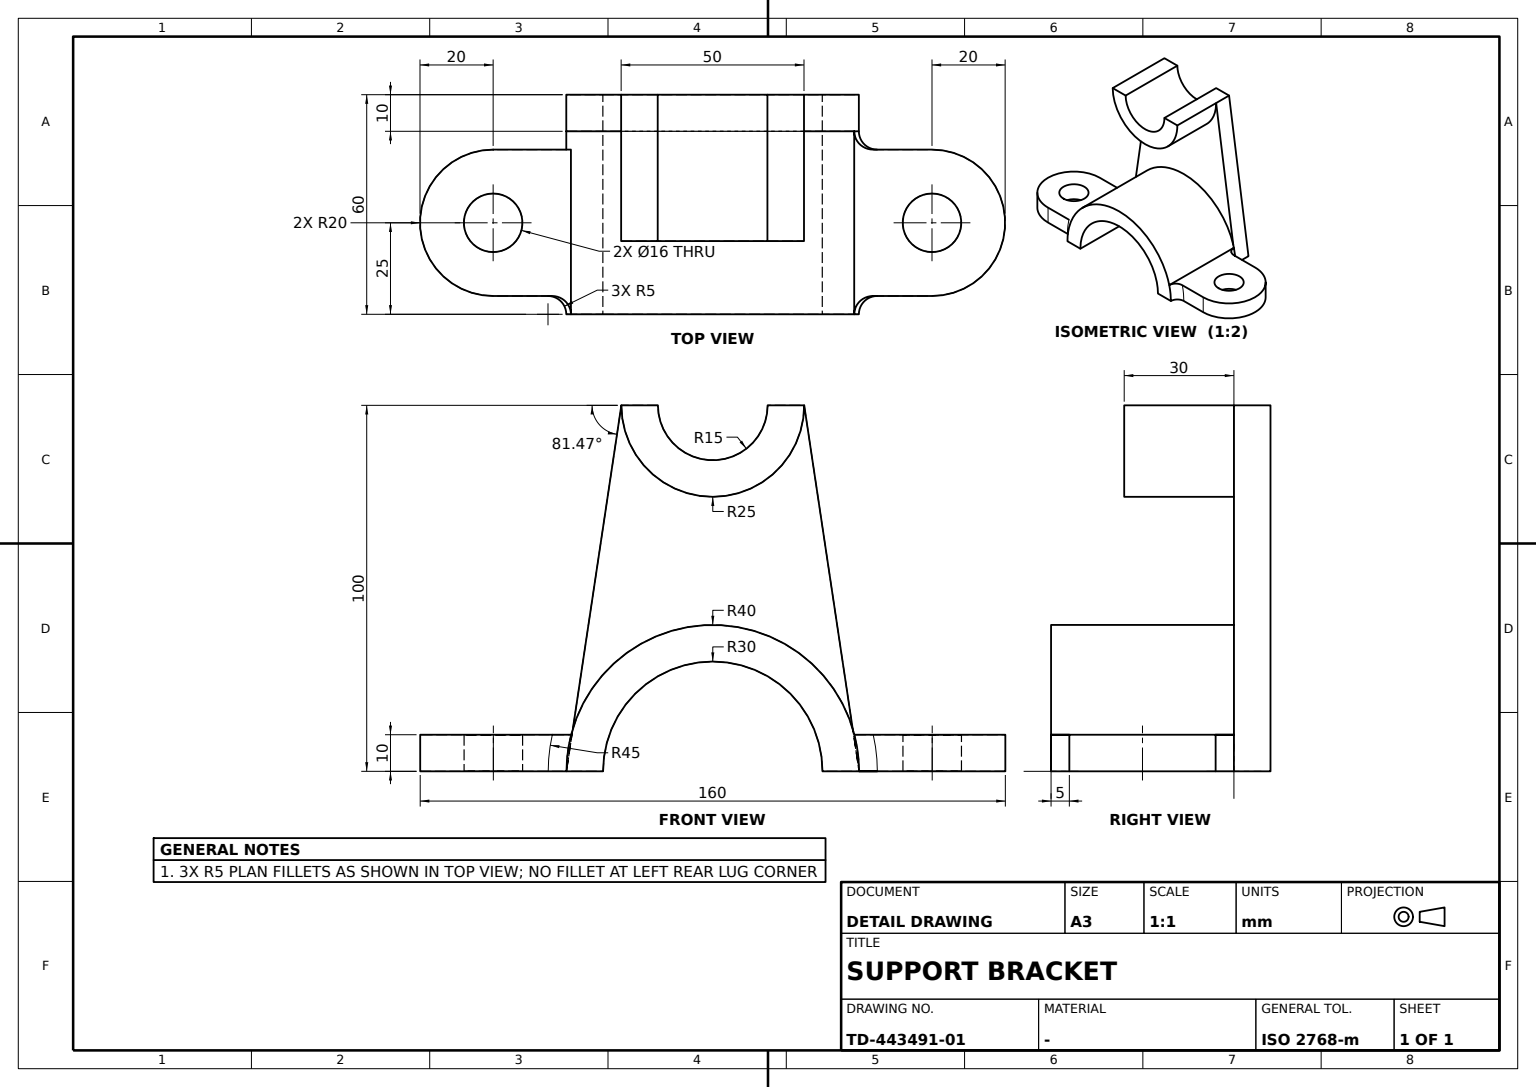
ISO-10303-21;
HEADER;
FILE_DESCRIPTION((''),'2;1');
FILE_NAME('','',(''),(''),'','','');
FILE_SCHEMA(('AUTOMOTIVE_DESIGN'));
ENDSEC;
DATA;
#1=APPLICATION_CONTEXT('');
#2=PRODUCT_CONTEXT('',#1,'mechanical');
#3=PRODUCT('','','',(#2));
#4=PRODUCT_DEFINITION_FORMATION('','',#3);
#5=PRODUCT_DEFINITION_CONTEXT('',#1,'design');
#6=PRODUCT_DEFINITION('','',#4,#5);
#7=PRODUCT_DEFINITION_SHAPE('','',#6);
#8=(LENGTH_UNIT()NAMED_UNIT(*)SI_UNIT(.MILLI.,.METRE.));
#9=(NAMED_UNIT(*)PLANE_ANGLE_UNIT()SI_UNIT($,.RADIAN.));
#10=(NAMED_UNIT(*)SI_UNIT($,.STERADIAN.)SOLID_ANGLE_UNIT());
#11=UNCERTAINTY_MEASURE_WITH_UNIT(LENGTH_MEASURE(0.005),#8,'distance_accuracy_value','');
#12=(GEOMETRIC_REPRESENTATION_CONTEXT(3)GLOBAL_UNCERTAINTY_ASSIGNED_CONTEXT((#11))GLOBAL_UNIT_ASSIGNED_CONTEXT((#8,#9,#10))REPRESENTATION_CONTEXT('',''));
#13=CARTESIAN_POINT('',(-8.,-60.,0.));
#14=VERTEX_POINT('',#13);
#15=CARTESIAN_POINT('',(0.,-60.,0.));
#16=DIRECTION('',(0.,0.,-1.));
#17=DIRECTION('',(-1.,0.,0.));
#18=AXIS2_PLACEMENT_3D('',#15,#16,#17);
#19=CIRCLE('',#18,8.);
#20=EDGE_CURVE('',#14,#14,#19,.T.);
#21=ORIENTED_EDGE('',*,*,#20,.T.);
#22=EDGE_LOOP('',(#21));
#23=FACE_BOUND('',#22,.T.);
#24=CARTESIAN_POINT('',(8.,-60.,10.));
#25=VERTEX_POINT('',#24);
#26=CARTESIAN_POINT('',(0.,-60.,10.));
#27=DIRECTION('',(0.,0.,1.));
#28=DIRECTION('',(1.,0.,0.));
#29=AXIS2_PLACEMENT_3D('',#26,#27,#28);
#30=CIRCLE('',#29,8.);
#31=EDGE_CURVE('',#25,#25,#30,.F.);
#32=ORIENTED_EDGE('',*,*,#31,.F.);
#33=EDGE_LOOP('',(#32));
#34=FACE_BOUND('',#33,.T.);
#35=CARTESIAN_POINT('',(0.,-60.,5.));
#36=AXIS2_PLACEMENT_3D('',#35,#16,#28);
#37=CYLINDRICAL_SURFACE('',#36,8.);
#38=ADVANCED_FACE('',(#23,#34),#37,.F.);
#39=CARTESIAN_POINT('',(20.,-45.,0.));
#40=VERTEX_POINT('',#39);
#41=CARTESIAN_POINT('',(25.,-40.,0.));
#42=VERTEX_POINT('',#41);
#43=CARTESIAN_POINT('',(25.,-45.,0.));
#44=AXIS2_PLACEMENT_3D('',#43,#16,#17);
#45=CIRCLE('',#44,5.);
#46=EDGE_CURVE('',#40,#42,#45,.T.);
#47=ORIENTED_EDGE('',*,*,#46,.F.);
#48=CARTESIAN_POINT('',(20.,-60.,0.));
#49=VERTEX_POINT('',#48);
#50=CARTESIAN_POINT('',(20.,40.,0.));
#51=DIRECTION('',(0.,-1.,0.));
#52=VECTOR('',#51,1000.);
#53=LINE('',#50,#52);
#54=EDGE_CURVE('',#40,#49,#53,.T.);
#55=ORIENTED_EDGE('',*,*,#54,.T.);
#56=CARTESIAN_POINT('',(-20.,-60.,0.));
#57=VERTEX_POINT('',#56);
#58=CIRCLE('',#18,20.);
#59=EDGE_CURVE('',#49,#57,#58,.T.);
#60=ORIENTED_EDGE('',*,*,#59,.T.);
#61=CARTESIAN_POINT('',(-20.,-40.,0.));
#62=VERTEX_POINT('',#61);
#63=CARTESIAN_POINT('',(-20.,40.,0.));
#64=DIRECTION('',(0.,1.,0.));
#65=VECTOR('',#64,1000.);
#66=LINE('',#63,#65);
#67=EDGE_CURVE('',#57,#62,#66,.T.);
#68=ORIENTED_EDGE('',*,*,#67,.T.);
#69=CARTESIAN_POINT('',(-25.,-40.,0.));
#70=VERTEX_POINT('',#69);
#71=VECTOR('',#17,1000.);
#72=LINE('',#61,#71);
#73=EDGE_CURVE('',#62,#70,#72,.T.);
#74=ORIENTED_EDGE('',*,*,#73,.T.);
#75=CARTESIAN_POINT('',(-35.,-40.,0.));
#76=VERTEX_POINT('',#75);
#77=LINE('',#69,#71);
#78=EDGE_CURVE('',#70,#76,#77,.T.);
#79=ORIENTED_EDGE('',*,*,#78,.T.);
#80=CARTESIAN_POINT('',(-35.,-30.,0.));
#81=VERTEX_POINT('',#80);
#82=CARTESIAN_POINT('',(-35.,0.,0.));
#83=LINE('',#82,#52);
#84=EDGE_CURVE('',#81,#76,#83,.T.);
#85=ORIENTED_EDGE('',*,*,#84,.F.);
#86=CARTESIAN_POINT('',(25.,-30.,0.));
#87=VERTEX_POINT('',#86);
#88=LINE('',#86,#71);
#89=EDGE_CURVE('',#87,#81,#88,.T.);
#90=ORIENTED_EDGE('',*,*,#89,.F.);
#91=CARTESIAN_POINT('',(25.,0.,0.));
#92=LINE('',#91,#52);
#93=EDGE_CURVE('',#87,#42,#92,.T.);
#94=ORIENTED_EDGE('',*,*,#93,.T.);
#95=EDGE_LOOP('',(#47,#55,#60,#68,#74,#79,#85,#90,#94));
#96=FACE_BOUND('',#95,.T.);
#97=ORIENTED_EDGE('',*,*,#20,.F.);
#98=EDGE_LOOP('',(#97));
#99=FACE_BOUND('',#98,.T.);
#100=CARTESIAN_POINT('',(0.,40.,0.));
#101=AXIS2_PLACEMENT_3D('',#100,#16,#51);
#102=PLANE('',#101);
#103=ADVANCED_FACE('',(#96,#99),#102,.T.);
#104=CARTESIAN_POINT('',(-25.,40.,0.));
#105=VERTEX_POINT('',#104);
#106=CARTESIAN_POINT('',(-25.,38.239609,11.735941));
#107=VERTEX_POINT('',#106);
#108=CARTESIAN_POINT('',(-25.,39.119804,5.867971));
#109=DIRECTION('',(0.,-0.148340453,0.988936353));
#110=VECTOR('',#109,1000.);
#111=LINE('',#108,#110);
#112=EDGE_CURVE('',#105,#107,#111,.T.);
#113=ORIENTED_EDGE('',*,*,#112,.T.);
#114=CARTESIAN_POINT('',(-25.,38.729833,10.));
#115=VERTEX_POINT('',#114);
#116=CARTESIAN_POINT('',(-25.,0.,0.));
#117=AXIS2_PLACEMENT_3D('',#116,#17,#27);
#118=CIRCLE('',#117,40.);
#119=EDGE_CURVE('',#107,#115,#118,.T.);
#120=ORIENTED_EDGE('',*,*,#119,.T.);
#121=EDGE_CURVE('',#115,#105,#118,.T.);
#122=ORIENTED_EDGE('',*,*,#121,.T.);
#123=EDGE_LOOP('',(#113,#120,#122));
#124=FACE_BOUND('',#123,.T.);
#125=AXIS2_PLACEMENT_3D('',#116,#17,#51);
#126=PLANE('',#125);
#127=ADVANCED_FACE('',(#124),#126,.T.);
#128=CARTESIAN_POINT('',(5.,-15.,100.));
#129=VERTEX_POINT('',#128);
#130=CARTESIAN_POINT('',(-35.,-15.,100.));
#131=VERTEX_POINT('',#130);
#132=VECTOR('',#28,1000.);
#133=LINE('',#128,#132);
#134=EDGE_CURVE('',#129,#131,#133,.F.);
#135=ORIENTED_EDGE('',*,*,#134,.T.);
#136=CARTESIAN_POINT('',(-35.,-25.,100.));
#137=VERTEX_POINT('',#136);
#138=CARTESIAN_POINT('',(-35.,0.,100.));
#139=LINE('',#138,#52);
#140=EDGE_CURVE('',#131,#137,#139,.T.);
#141=ORIENTED_EDGE('',*,*,#140,.T.);
#142=CARTESIAN_POINT('',(-25.,-25.,100.));
#143=VERTEX_POINT('',#142);
#144=LINE('',#142,#71);
#145=EDGE_CURVE('',#143,#137,#144,.T.);
#146=ORIENTED_EDGE('',*,*,#145,.F.);
#147=CARTESIAN_POINT('',(5.,-25.,100.));
#148=VERTEX_POINT('',#147);
#149=LINE('',#142,#132);
#150=EDGE_CURVE('',#143,#148,#149,.T.);
#151=ORIENTED_EDGE('',*,*,#150,.T.);
#152=CARTESIAN_POINT('',(5.,0.,100.));
#153=LINE('',#152,#65);
#154=EDGE_CURVE('',#148,#129,#153,.T.);
#155=ORIENTED_EDGE('',*,*,#154,.T.);
#156=EDGE_LOOP('',(#135,#141,#146,#151,#155));
#157=FACE_BOUND('',#156,.T.);
#158=CARTESIAN_POINT('',(-25.,25.,100.));
#159=AXIS2_PLACEMENT_3D('',#158,#16,#51);
#160=PLANE('',#159);
#161=ADVANCED_FACE('',(#157),#160,.F.);
#162=CARTESIAN_POINT('',(-35.,15.,100.));
#163=VERTEX_POINT('',#162);
#164=AXIS2_PLACEMENT_3D('',#138,#17,#27);
#165=CIRCLE('',#164,15.);
#166=EDGE_CURVE('',#163,#131,#165,.T.);
#167=ORIENTED_EDGE('',*,*,#166,.T.);
#168=ORIENTED_EDGE('',*,*,#134,.F.);
#169=CARTESIAN_POINT('',(5.,15.,100.));
#170=VERTEX_POINT('',#169);
#171=AXIS2_PLACEMENT_3D('',#152,#28,#16);
#172=CIRCLE('',#171,15.);
#173=EDGE_CURVE('',#129,#170,#172,.T.);
#174=ORIENTED_EDGE('',*,*,#173,.T.);
#175=LINE('',#169,#132);
#176=EDGE_CURVE('',#170,#163,#175,.F.);
#177=ORIENTED_EDGE('',*,*,#176,.T.);
#178=EDGE_LOOP('',(#167,#168,#174,#177));
#179=FACE_BOUND('',#178,.T.);
#180=CARTESIAN_POINT('',(-10.,0.,100.));
#181=AXIS2_PLACEMENT_3D('',#180,#28,#64);
#182=CYLINDRICAL_SURFACE('',#181,15.);
#183=ADVANCED_FACE('',(#179),#182,.F.);
#184=CARTESIAN_POINT('',(20.,45.,0.));
#185=VERTEX_POINT('',#184);
#186=CARTESIAN_POINT('',(20.,60.,0.));
#187=VERTEX_POINT('',#186);
#188=CARTESIAN_POINT('',(20.,38.,0.));
#189=LINE('',#188,#65);
#190=EDGE_CURVE('',#185,#187,#189,.T.);
#191=ORIENTED_EDGE('',*,*,#190,.T.);
#192=CARTESIAN_POINT('',(20.,60.,10.));
#193=VERTEX_POINT('',#192);
#194=CARTESIAN_POINT('',(20.,60.,5.));
#195=VECTOR('',#27,1000.);
#196=LINE('',#194,#195);
#197=EDGE_CURVE('',#187,#193,#196,.T.);
#198=ORIENTED_EDGE('',*,*,#197,.T.);
#199=CARTESIAN_POINT('',(20.,43.874822,10.));
#200=VERTEX_POINT('',#199);
#201=CARTESIAN_POINT('',(20.,0.,10.));
#202=LINE('',#201,#65);
#203=EDGE_CURVE('',#200,#193,#202,.T.);
#204=ORIENTED_EDGE('',*,*,#203,.F.);
#205=CARTESIAN_POINT('',(20.,0.,0.));
#206=AXIS2_PLACEMENT_3D('',#205,#28,#16);
#207=CIRCLE('',#206,45.);
#208=EDGE_CURVE('',#185,#200,#207,.T.);
#209=ORIENTED_EDGE('',*,*,#208,.F.);
#210=EDGE_LOOP('',(#191,#198,#204,#209));
#211=FACE_BOUND('',#210,.T.);
#212=AXIS2_PLACEMENT_3D('',#188,#28,#64);
#213=PLANE('',#212);
#214=ADVANCED_FACE('',(#211),#213,.T.);
#215=CARTESIAN_POINT('',(-35.,40.,0.));
#216=VERTEX_POINT('',#215);
#217=LINE('',#100,#71);
#218=EDGE_CURVE('',#105,#216,#217,.T.);
#219=ORIENTED_EDGE('',*,*,#218,.T.);
#220=CARTESIAN_POINT('',(-35.,25.,100.));
#221=VERTEX_POINT('',#220);
#222=CARTESIAN_POINT('',(-35.,39.119804,5.867971));
#223=LINE('',#222,#110);
#224=EDGE_CURVE('',#216,#221,#223,.T.);
#225=ORIENTED_EDGE('',*,*,#224,.T.);
#226=VERTEX_POINT('',#158);
#227=LINE('',#158,#71);
#228=EDGE_CURVE('',#226,#221,#227,.T.);
#229=ORIENTED_EDGE('',*,*,#228,.F.);
#230=EDGE_CURVE('',#107,#226,#111,.T.);
#231=ORIENTED_EDGE('',*,*,#230,.F.);
#232=ORIENTED_EDGE('',*,*,#112,.F.);
#233=EDGE_LOOP('',(#219,#225,#229,#231,#232));
#234=FACE_BOUND('',#233,.T.);
#235=DIRECTION('',(0.,-0.988936353,-0.148340453));
#236=AXIS2_PLACEMENT_3D('',#104,#235,#109);
#237=PLANE('',#236);
#238=ADVANCED_FACE('',(#234),#237,.F.);
#239=ORIENTED_EDGE('',*,*,#31,.T.);
#240=EDGE_LOOP('',(#239));
#241=FACE_BOUND('',#240,.T.);
#242=CARTESIAN_POINT('',(-20.,-60.,10.));
#243=VERTEX_POINT('',#242);
#244=CARTESIAN_POINT('',(-20.,-38.729833,10.));
#245=VERTEX_POINT('',#244);
#246=CARTESIAN_POINT('',(-20.,60.,10.));
#247=LINE('',#246,#65);
#248=EDGE_CURVE('',#243,#245,#247,.T.);
#249=ORIENTED_EDGE('',*,*,#248,.F.);
#250=CARTESIAN_POINT('',(20.,-60.,10.));
#251=VERTEX_POINT('',#250);
#252=CIRCLE('',#29,20.);
#253=EDGE_CURVE('',#251,#243,#252,.F.);
#254=ORIENTED_EDGE('',*,*,#253,.F.);
#255=CARTESIAN_POINT('',(20.,-43.874825,10.));
#256=VERTEX_POINT('',#255);
#257=CARTESIAN_POINT('',(20.,38.,10.));
#258=LINE('',#257,#52);
#259=EDGE_CURVE('',#256,#251,#258,.T.);
#260=ORIENTED_EDGE('',*,*,#259,.F.);
#261=CARTESIAN_POINT('',(25.,-38.729833,10.));
#262=VERTEX_POINT('',#261);
#263=CARTESIAN_POINT('',(19.999999,-42.535505,10.));
#264=CARTESIAN_POINT('',(21.050222,-39.899186,10.));
#265=CARTESIAN_POINT('',(23.659591,-38.729833,10.));
#266=B_SPLINE_CURVE_WITH_KNOTS('',3,(#255,#263,#264,#265,#261),.UNSPECIFIED.,.F.,.F.,(4,1,4),(0.000000003,0.003961233,0.007922464),.UNSPECIFIED.);
#267=EDGE_CURVE('',#256,#262,#266,.T.);
#268=ORIENTED_EDGE('',*,*,#267,.T.);
#269=LINE('',#244,#71);
#270=EDGE_CURVE('',#245,#262,#269,.F.);
#271=ORIENTED_EDGE('',*,*,#270,.F.);
#272=EDGE_LOOP('',(#249,#254,#260,#268,#271));
#273=FACE_BOUND('',#272,.T.);
#274=CARTESIAN_POINT('',(0.,0.,10.));
#275=AXIS2_PLACEMENT_3D('',#274,#27,#28);
#276=PLANE('',#275);
#277=ADVANCED_FACE('',(#241,#273),#276,.T.);
#278=CARTESIAN_POINT('',(-20.,45.,0.));
#279=VERTEX_POINT('',#278);
#280=CARTESIAN_POINT('',(-25.,45.,0.));
#281=AXIS2_PLACEMENT_3D('',#280,#16,#17);
#282=CIRCLE('',#281,5.);
#283=EDGE_CURVE('',#279,#105,#282,.T.);
#284=ORIENTED_EDGE('',*,*,#283,.T.);
#285=ORIENTED_EDGE('',*,*,#121,.F.);
#286=CARTESIAN_POINT('',(-20.,43.874822,10.));
#287=VERTEX_POINT('',#286);
#288=CARTESIAN_POINT('',(-20.,42.535503,10.));
#289=CARTESIAN_POINT('',(-21.050223,39.899185,10.));
#290=CARTESIAN_POINT('',(-23.659592,38.729833,10.));
#291=B_SPLINE_CURVE_WITH_KNOTS('',3,(#286,#288,#289,#290,#114),.UNSPECIFIED.,.F.,.F.,(4,1,4),(0.,0.003961229,0.007922459),.UNSPECIFIED.);
#292=EDGE_CURVE('',#287,#115,#291,.T.);
#293=ORIENTED_EDGE('',*,*,#292,.F.);
#294=CARTESIAN_POINT('',(-20.,0.,0.));
#295=AXIS2_PLACEMENT_3D('',#294,#17,#27);
#296=CIRCLE('',#295,45.);
#297=EDGE_CURVE('',#287,#279,#296,.T.);
#298=ORIENTED_EDGE('',*,*,#297,.T.);
#299=EDGE_LOOP('',(#284,#285,#293,#298));
#300=FACE_BOUND('',#299,.T.);
#301=DIRECTION('',(0.,-0.539755066,-0.841822112));
#302=AXIS2_PLACEMENT_3D('',#116,#17,#301);
#303=TOROIDAL_SURFACE('',#302,45.,5.);
#304=ADVANCED_FACE('',(#300),#303,.F.);
#305=CARTESIAN_POINT('',(-35.,30.,0.));
#306=VERTEX_POINT('',#305);
#307=AXIS2_PLACEMENT_3D('',#82,#17,#27);
#308=CIRCLE('',#307,30.);
#309=EDGE_CURVE('',#81,#306,#308,.T.);
#310=ORIENTED_EDGE('',*,*,#309,.T.);
#311=CARTESIAN_POINT('',(25.,30.,0.));
#312=VERTEX_POINT('',#311);
#313=LINE('',#311,#71);
#314=EDGE_CURVE('',#312,#306,#313,.T.);
#315=ORIENTED_EDGE('',*,*,#314,.F.);
#316=AXIS2_PLACEMENT_3D('',#91,#17,#27);
#317=CIRCLE('',#316,30.);
#318=EDGE_CURVE('',#87,#312,#317,.T.);
#319=ORIENTED_EDGE('',*,*,#318,.F.);
#320=ORIENTED_EDGE('',*,*,#89,.T.);
#321=EDGE_LOOP('',(#310,#315,#319,#320));
#322=FACE_BOUND('',#321,.T.);
#323=CARTESIAN_POINT('',(0.,0.,0.));
#324=AXIS2_PLACEMENT_3D('',#323,#17,#51);
#325=CYLINDRICAL_SURFACE('',#324,30.);
#326=ADVANCED_FACE('',(#322),#325,.F.);
#327=ORIENTED_EDGE('',*,*,#166,.F.);
#328=EDGE_CURVE('',#221,#163,#139,.T.);
#329=ORIENTED_EDGE('',*,*,#328,.F.);
#330=ORIENTED_EDGE('',*,*,#224,.F.);
#331=EDGE_CURVE('',#216,#306,#83,.T.);
#332=ORIENTED_EDGE('',*,*,#331,.T.);
#333=ORIENTED_EDGE('',*,*,#309,.F.);
#334=ORIENTED_EDGE('',*,*,#84,.T.);
#335=CARTESIAN_POINT('',(-35.,-39.119804,5.867971));
#336=DIRECTION('',(0.,-0.148340453,-0.988936353));
#337=VECTOR('',#336,1000.);
#338=LINE('',#335,#337);
#339=EDGE_CURVE('',#137,#76,#338,.T.);
#340=ORIENTED_EDGE('',*,*,#339,.F.);
#341=ORIENTED_EDGE('',*,*,#140,.F.);
#342=EDGE_LOOP('',(#327,#329,#330,#332,#333,#334,#340,#341));
#343=FACE_BOUND('',#342,.T.);
#344=AXIS2_PLACEMENT_3D('',#82,#17,#51);
#345=PLANE('',#344);
#346=ADVANCED_FACE('',(#343),#345,.T.);
#347=CARTESIAN_POINT('',(5.,25.,100.));
#348=VERTEX_POINT('',#347);
#349=EDGE_CURVE('',#170,#348,#153,.T.);
#350=ORIENTED_EDGE('',*,*,#349,.F.);
#351=ORIENTED_EDGE('',*,*,#173,.F.);
#352=ORIENTED_EDGE('',*,*,#154,.F.);
#353=CIRCLE('',#171,25.);
#354=EDGE_CURVE('',#148,#348,#353,.T.);
#355=ORIENTED_EDGE('',*,*,#354,.T.);
#356=EDGE_LOOP('',(#350,#351,#352,#355));
#357=FACE_BOUND('',#356,.T.);
#358=CARTESIAN_POINT('',(5.,0.,0.));
#359=AXIS2_PLACEMENT_3D('',#358,#28,#64);
#360=PLANE('',#359);
#361=ADVANCED_FACE('',(#357),#360,.T.);
#362=CARTESIAN_POINT('',(-25.,-38.239609,11.735941));
#363=VERTEX_POINT('',#362);
#364=EDGE_CURVE('',#70,#363,#118,.T.);
#365=ORIENTED_EDGE('',*,*,#364,.T.);
#366=CARTESIAN_POINT('',(-25.,-39.119804,5.867971));
#367=LINE('',#366,#337);
#368=EDGE_CURVE('',#363,#70,#367,.T.);
#369=ORIENTED_EDGE('',*,*,#368,.T.);
#370=EDGE_LOOP('',(#365,#369));
#371=FACE_BOUND('',#370,.T.);
#372=ADVANCED_FACE('',(#371),#126,.T.);
#373=ORIENTED_EDGE('',*,*,#248,.T.);
#374=CIRCLE('',#295,40.);
#375=EDGE_CURVE('',#62,#245,#374,.T.);
#376=ORIENTED_EDGE('',*,*,#375,.F.);
#377=ORIENTED_EDGE('',*,*,#67,.F.);
#378=CARTESIAN_POINT('',(-20.,-60.,5.));
#379=VECTOR('',#16,1000.);
#380=LINE('',#378,#379);
#381=EDGE_CURVE('',#57,#243,#380,.F.);
#382=ORIENTED_EDGE('',*,*,#381,.T.);
#383=EDGE_LOOP('',(#373,#376,#377,#382));
#384=FACE_BOUND('',#383,.T.);
#385=CARTESIAN_POINT('',(-20.,60.,0.));
#386=AXIS2_PLACEMENT_3D('',#385,#17,#51);
#387=PLANE('',#386);
#388=ADVANCED_FACE('',(#384),#387,.T.);
#389=EDGE_CURVE('',#143,#363,#367,.T.);
#390=ORIENTED_EDGE('',*,*,#389,.F.);
#391=ORIENTED_EDGE('',*,*,#145,.T.);
#392=ORIENTED_EDGE('',*,*,#339,.T.);
#393=ORIENTED_EDGE('',*,*,#78,.F.);
#394=ORIENTED_EDGE('',*,*,#368,.F.);
#395=EDGE_LOOP('',(#390,#391,#392,#393,#394));
#396=FACE_BOUND('',#395,.T.);
#397=DIRECTION('',(0.,0.988936353,-0.148340453));
#398=AXIS2_PLACEMENT_3D('',#142,#397,#336);
#399=PLANE('',#398);
#400=ADVANCED_FACE('',(#396),#399,.F.);
#401=CARTESIAN_POINT('',(-25.,0.,100.));
#402=AXIS2_PLACEMENT_3D('',#401,#17,#27);
#403=CIRCLE('',#402,25.);
#404=EDGE_CURVE('',#143,#226,#403,.F.);
#405=ORIENTED_EDGE('',*,*,#404,.F.);
#406=ORIENTED_EDGE('',*,*,#389,.T.);
#407=EDGE_CURVE('',#363,#107,#118,.T.);
#408=ORIENTED_EDGE('',*,*,#407,.T.);
#409=ORIENTED_EDGE('',*,*,#230,.T.);
#410=EDGE_LOOP('',(#405,#406,#408,#409));
#411=FACE_BOUND('',#410,.T.);
#412=ADVANCED_FACE('',(#411),#126,.F.);
#413=ORIENTED_EDGE('',*,*,#404,.T.);
#414=LINE('',#158,#132);
#415=EDGE_CURVE('',#226,#348,#414,.T.);
#416=ORIENTED_EDGE('',*,*,#415,.T.);
#417=ORIENTED_EDGE('',*,*,#354,.F.);
#418=ORIENTED_EDGE('',*,*,#150,.F.);
#419=EDGE_LOOP('',(#413,#416,#417,#418));
#420=FACE_BOUND('',#419,.T.);
#421=CYLINDRICAL_SURFACE('',#181,25.);
#422=ADVANCED_FACE('',(#420),#421,.T.);
#423=AXIS2_PLACEMENT_3D('',#91,#28,#16);
#424=CIRCLE('',#423,40.);
#425=EDGE_CURVE('',#42,#262,#424,.F.);
#426=ORIENTED_EDGE('',*,*,#425,.F.);
#427=ORIENTED_EDGE('',*,*,#93,.F.);
#428=ORIENTED_EDGE('',*,*,#318,.T.);
#429=CARTESIAN_POINT('',(25.,40.,0.));
#430=VERTEX_POINT('',#429);
#431=EDGE_CURVE('',#430,#312,#92,.T.);
#432=ORIENTED_EDGE('',*,*,#431,.F.);
#433=CARTESIAN_POINT('',(25.,38.729833,10.));
#434=VERTEX_POINT('',#433);
#435=EDGE_CURVE('',#434,#430,#424,.F.);
#436=ORIENTED_EDGE('',*,*,#435,.F.);
#437=CIRCLE('',#316,40.);
#438=EDGE_CURVE('',#262,#434,#437,.T.);
#439=ORIENTED_EDGE('',*,*,#438,.F.);
#440=EDGE_LOOP('',(#426,#427,#428,#432,#436,#439));
#441=FACE_BOUND('',#440,.T.);
#442=AXIS2_PLACEMENT_3D('',#91,#17,#51);
#443=PLANE('',#442);
#444=ADVANCED_FACE('',(#441),#443,.F.);
#445=ORIENTED_EDGE('',*,*,#208,.T.);
#446=CARTESIAN_POINT('',(20.,42.535503,10.));
#447=CARTESIAN_POINT('',(21.050223,39.899185,10.));
#448=CARTESIAN_POINT('',(23.659592,38.729833,10.));
#449=B_SPLINE_CURVE_WITH_KNOTS('',3,(#199,#446,#447,#448,#433),.UNSPECIFIED.,.F.,.F.,(4,1,4),(0.,0.003961229,0.007922459),.UNSPECIFIED.);
#450=EDGE_CURVE('',#200,#434,#449,.T.);
#451=ORIENTED_EDGE('',*,*,#450,.T.);
#452=ORIENTED_EDGE('',*,*,#435,.T.);
#453=CARTESIAN_POINT('',(25.,45.,0.));
#454=AXIS2_PLACEMENT_3D('',#453,#16,#17);
#455=CIRCLE('',#454,5.);
#456=EDGE_CURVE('',#185,#430,#455,.F.);
#457=ORIENTED_EDGE('',*,*,#456,.F.);
#458=EDGE_LOOP('',(#445,#451,#452,#457));
#459=FACE_BOUND('',#458,.T.);
#460=DIRECTION('',(0.,0.488366621,-0.872638553));
#461=AXIS2_PLACEMENT_3D('',#91,#28,#460);
#462=TOROIDAL_SURFACE('',#461,45.,5.);
#463=ADVANCED_FACE('',(#459),#462,.F.);
#464=ORIENTED_EDGE('',*,*,#425,.T.);
#465=ORIENTED_EDGE('',*,*,#267,.F.);
#466=EDGE_CURVE('',#256,#40,#207,.T.);
#467=ORIENTED_EDGE('',*,*,#466,.T.);
#468=ORIENTED_EDGE('',*,*,#46,.T.);
#469=EDGE_LOOP('',(#464,#465,#467,#468));
#470=FACE_BOUND('',#469,.T.);
#471=ADVANCED_FACE('',(#470),#462,.F.);
#472=VERTEX_POINT('',#246);
#473=CARTESIAN_POINT('',(-20.,0.,10.));
#474=LINE('',#473,#52);
#475=EDGE_CURVE('',#472,#287,#474,.T.);
#476=ORIENTED_EDGE('',*,*,#475,.F.);
#477=VERTEX_POINT('',#385);
#478=CARTESIAN_POINT('',(-20.,60.,5.));
#479=LINE('',#478,#195);
#480=EDGE_CURVE('',#477,#472,#479,.T.);
#481=ORIENTED_EDGE('',*,*,#480,.F.);
#482=LINE('',#385,#52);
#483=EDGE_CURVE('',#477,#279,#482,.T.);
#484=ORIENTED_EDGE('',*,*,#483,.T.);
#485=ORIENTED_EDGE('',*,*,#297,.F.);
#486=EDGE_LOOP('',(#476,#481,#484,#485));
#487=FACE_BOUND('',#486,.T.);
#488=ADVANCED_FACE('',(#487),#387,.T.);
#489=ORIENTED_EDGE('',*,*,#54,.F.);
#490=ORIENTED_EDGE('',*,*,#466,.F.);
#491=ORIENTED_EDGE('',*,*,#259,.T.);
#492=CARTESIAN_POINT('',(20.,-60.,5.));
#493=LINE('',#492,#379);
#494=EDGE_CURVE('',#49,#251,#493,.F.);
#495=ORIENTED_EDGE('',*,*,#494,.F.);
#496=EDGE_LOOP('',(#489,#490,#491,#495));
#497=FACE_BOUND('',#496,.T.);
#498=ADVANCED_FACE('',(#497),#213,.T.);
#499=ORIENTED_EDGE('',*,*,#475,.T.);
#500=ORIENTED_EDGE('',*,*,#292,.T.);
#501=LINE('',#433,#71);
#502=EDGE_CURVE('',#434,#115,#501,.T.);
#503=ORIENTED_EDGE('',*,*,#502,.F.);
#504=ORIENTED_EDGE('',*,*,#450,.F.);
#505=ORIENTED_EDGE('',*,*,#203,.T.);
#506=CARTESIAN_POINT('',(0.,60.,10.));
#507=AXIS2_PLACEMENT_3D('',#506,#27,#28);
#508=CIRCLE('',#507,20.);
#509=EDGE_CURVE('',#193,#472,#508,.T.);
#510=ORIENTED_EDGE('',*,*,#509,.T.);
#511=EDGE_LOOP('',(#499,#500,#503,#504,#505,#510));
#512=FACE_BOUND('',#511,.T.);
#513=CARTESIAN_POINT('',(8.,60.,10.));
#514=VERTEX_POINT('',#513);
#515=CIRCLE('',#507,8.);
#516=EDGE_CURVE('',#514,#514,#515,.T.);
#517=ORIENTED_EDGE('',*,*,#516,.F.);
#518=EDGE_LOOP('',(#517));
#519=FACE_BOUND('',#518,.T.);
#520=ADVANCED_FACE('',(#512,#519),#276,.T.);
#521=ORIENTED_EDGE('',*,*,#59,.F.);
#522=ORIENTED_EDGE('',*,*,#494,.T.);
#523=ORIENTED_EDGE('',*,*,#253,.T.);
#524=ORIENTED_EDGE('',*,*,#381,.F.);
#525=EDGE_LOOP('',(#521,#522,#523,#524));
#526=FACE_BOUND('',#525,.T.);
#527=CYLINDRICAL_SURFACE('',#36,20.);
#528=ADVANCED_FACE('',(#526),#527,.T.);
#529=ORIENTED_EDGE('',*,*,#375,.T.);
#530=ORIENTED_EDGE('',*,*,#270,.T.);
#531=ORIENTED_EDGE('',*,*,#438,.T.);
#532=ORIENTED_EDGE('',*,*,#502,.T.);
#533=ORIENTED_EDGE('',*,*,#119,.F.);
#534=ORIENTED_EDGE('',*,*,#407,.F.);
#535=ORIENTED_EDGE('',*,*,#364,.F.);
#536=ORIENTED_EDGE('',*,*,#73,.F.);
#537=EDGE_LOOP('',(#529,#530,#531,#532,#533,#534,#535,#536));
#538=FACE_BOUND('',#537,.T.);
#539=CYLINDRICAL_SURFACE('',#324,40.);
#540=ADVANCED_FACE('',(#538),#539,.T.);
#541=ORIENTED_EDGE('',*,*,#328,.T.);
#542=ORIENTED_EDGE('',*,*,#176,.F.);
#543=ORIENTED_EDGE('',*,*,#349,.T.);
#544=ORIENTED_EDGE('',*,*,#415,.F.);
#545=ORIENTED_EDGE('',*,*,#228,.T.);
#546=EDGE_LOOP('',(#541,#542,#543,#544,#545));
#547=FACE_BOUND('',#546,.T.);
#548=ADVANCED_FACE('',(#547),#160,.F.);
#549=ORIENTED_EDGE('',*,*,#509,.F.);
#550=ORIENTED_EDGE('',*,*,#197,.F.);
#551=CARTESIAN_POINT('',(0.,60.,0.));
#552=AXIS2_PLACEMENT_3D('',#551,#16,#17);
#553=CIRCLE('',#552,20.);
#554=EDGE_CURVE('',#187,#477,#553,.F.);
#555=ORIENTED_EDGE('',*,*,#554,.T.);
#556=ORIENTED_EDGE('',*,*,#480,.T.);
#557=EDGE_LOOP('',(#549,#550,#555,#556));
#558=FACE_BOUND('',#557,.T.);
#559=CARTESIAN_POINT('',(0.,60.,5.));
#560=AXIS2_PLACEMENT_3D('',#559,#27,#28);
#561=CYLINDRICAL_SURFACE('',#560,20.);
#562=ADVANCED_FACE('',(#558),#561,.T.);
#563=ORIENTED_EDGE('',*,*,#314,.T.);
#564=ORIENTED_EDGE('',*,*,#331,.F.);
#565=ORIENTED_EDGE('',*,*,#218,.F.);
#566=ORIENTED_EDGE('',*,*,#283,.F.);
#567=ORIENTED_EDGE('',*,*,#483,.F.);
#568=ORIENTED_EDGE('',*,*,#554,.F.);
#569=ORIENTED_EDGE('',*,*,#190,.F.);
#570=ORIENTED_EDGE('',*,*,#456,.T.);
#571=ORIENTED_EDGE('',*,*,#431,.T.);
#572=EDGE_LOOP('',(#563,#564,#565,#566,#567,#568,#569,#570,#571));
#573=FACE_BOUND('',#572,.T.);
#574=CARTESIAN_POINT('',(-8.,60.,0.));
#575=VERTEX_POINT('',#574);
#576=CIRCLE('',#552,8.);
#577=EDGE_CURVE('',#575,#575,#576,.F.);
#578=ORIENTED_EDGE('',*,*,#577,.T.);
#579=EDGE_LOOP('',(#578));
#580=FACE_BOUND('',#579,.T.);
#581=ADVANCED_FACE('',(#573,#580),#102,.T.);
#582=ORIENTED_EDGE('',*,*,#516,.T.);
#583=EDGE_LOOP('',(#582));
#584=FACE_BOUND('',#583,.T.);
#585=ORIENTED_EDGE('',*,*,#577,.F.);
#586=EDGE_LOOP('',(#585));
#587=FACE_BOUND('',#586,.T.);
#588=CYLINDRICAL_SURFACE('',#560,8.);
#589=ADVANCED_FACE('',(#584,#587),#588,.F.);
#590=CLOSED_SHELL('',(#38,#103,#127,#161,#183,#214,#238,#277,#304,#326,#346,#361,#372,#388,#400,#412,#422,#444,#463,#471,#488,#498,#520,#528,#540,#548,#562,#581,#589));
#591=MANIFOLD_SOLID_BREP('',#590);
#592=ADVANCED_BREP_SHAPE_REPRESENTATION('',(#591),#12);
#593=SHAPE_DEFINITION_REPRESENTATION(#7,#592);
ENDSEC;
END-ISO-10303-21;
